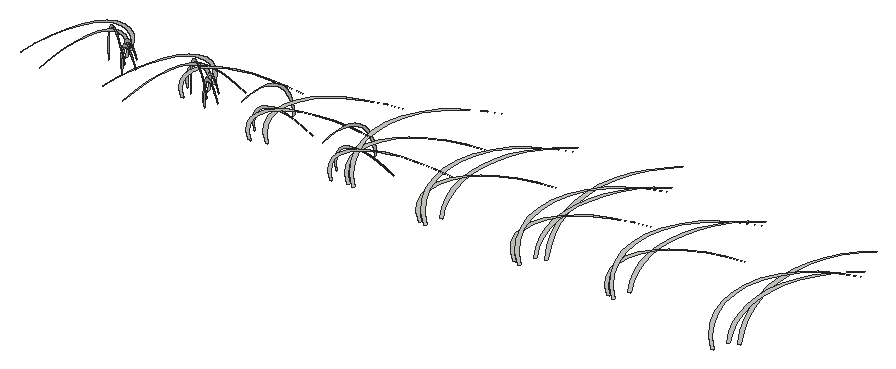
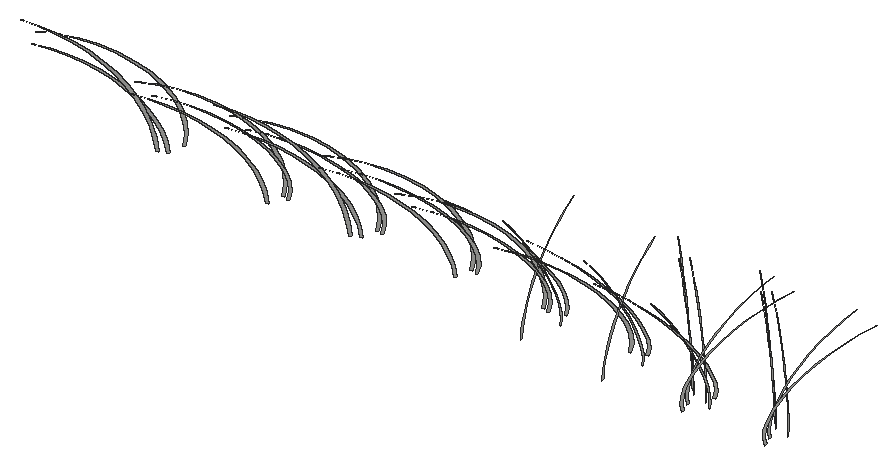
# SketchUp Ruby script. Lengths in inches.
U = 1.inch
M = Sketchup.active_model
def pt(a) = Geom::Point3d.new(a.map { |v| v * U })
def face(e, loops, mat)
  f = e.add_face(loops[0].map { |a| pt(a) })
  loops[1..].each { |l| e.add_face(l.map { |a| pt(a) }).erase! }
  f.material = f.back_material = mat if mat
  f
end
# faces: each face lists its corners as indices into pts; further lists are holes
def faces(e, pts, list, mat = nil) = list.each { |f| face(e, (f[0].is_a?(Array) ? f : [f]).map { |l| l.map { |i| pts[i] } }, mat) }
# xy, xz, yz: faces in a plane at the given z, y or x. An outline is a flat list of corners, or four numbers for a rectangle; further outlines are holes
def ring(l) = l.size == 4 ? [[l[0], l[1]], [l[2], l[1]], [l[2], l[3]], [l[0], l[3]]] : l.each_slice(2).to_a
def flat(e, list, mat, &to3) = list.each { |f| face(e, (f[0].is_a?(Array) ? f : [f]).map { |l| ring(l).map { |u, v| to3.(u, v) } }, mat) }
def xy(e, z, list, mat = nil) = flat(e, list, mat) { |x, y| [x, y, z] }
def xz(e, y, list, mat = nil) = flat(e, list, mat) { |x, z| [x, y, z] }
def yz(e, x, list, mat = nil) = flat(e, list, mat) { |y, z| [x, y, z] }
def lines(e, pts, list) = list.each { |a, b| e.add_line(pt(pts[a]), pt(pts[b])) }
# prism: a flat outline (further loops are holes) pulled along v
def prism(e, loops, v, mat = nil)
  f = face(e, loops, mat); d = Geom::Vector3d.new(v.map { |x| x * U })
  f.pushpull(f.normal.samedirection?(d) ? d.length : -d.length)
end
def box(e, o, s, mat = nil) = prism(e, [[o, [o[0] + s[0], o[1], o[2]], [o[0] + s[0], o[1] + s[1], o[2]], [o[0], o[1] + s[1], o[2]]]], [0, 0, s[2]], mat)
def at(x, y, z, deg = 0) = Geom::Transformation.translation(pt([x, y, z])) * Geom::Transformation.rotation(ORIGIN, Z_AXIS, deg.degrees)
def axes(o, x, y, z) = Geom::Transformation.new([*x, 0, *y, 0, *z, 0, *pt(o).to_a, 1])
def part(name) = M.definitions.add(name)
# library, detail: a bought-in or finely detailed component or shape, given as its bounding box
def library(name, o, s) = part(name).tap { |d| box(d.entities, o, s) }
def detail(e, o, s) = box(e.add_group.entities, o, s)
def put(e, d, t, mat = nil) = e.add_instance(d, t).tap { |i| i.material = mat if mat }
def group(e, t, mat = nil) = e.add_group.tap { |g| g.transformation = t; g.material = mat if mat }.entities
root = M.entities
g1 = group(root,at(402.8125,271.97,0))
p = [[0.125,-0.99,0],[0.06,-0.4375,0],[0,0,1.49],[0.02,-0.18,2.99],[0.12,-0.96,4.45],[0.3,-2.34,5.86],
  [0.54,-4.28,7.16],[0.85,-6.72,8.33],[1.21,-9.61,9.33],[1.62,-12.88,10.15],[2.07,-16.44,10.77],[2.55,-20.21,11.16],
  [3.03,-24.1,11.32],[3.53,-28,11.24],[3.04,-24.17,11.26],[2.57,-20.38,11.05],[2.11,-16.72,10.625],[1.67,-13.27,9.99],
  [1.27,-10.1,9.16],[0.92,-7.3,8.16],[0.62,-4.93,7.01],[0.38,-3.04,5.73],[0.21,-1.67,4.36],[0.11,-0.87,2.93],
  [0.08,-0.64,1.46]]
faces(g1,p,[[0,1,2,3,4,5,6,7,8,9,10,11,12,13,14,15,16,17,18,19,20,21,22,23,24]])
g2 = group(root,at(405.48,266.78,0))
p = [[14.61,-14.77,15.34],[16.8125,-17,15.75],[14.68,-14.84,15.26],[12.62,-12.76,14.58],[10.65,-10.77,13.72],[8.8,-8.9,12.69],
  [7.09,-7.17,11.5],[5.54,-5.61,10.16],[4.17,-4.22,8.7],[2.98,-3.02,7.11],[2,-2.02,5.43],[1.24,-1.25,3.67],
  [0.69,-0.7,1.86],[0.38,-0.38,0],[0,0,0],[0.26,-0.26,1.9],[0.77,-0.77,3.76],[1.52,-1.54,5.57],
  [2.51,-2.53,7.28],[3.72,-3.76,8.9],[5.13,-5.19,10.39],[6.74,-6.8125,11.73],[8.51,-8.61,12.91],[10.43,-10.55,13.91],
  [12.47,-12.61,14.73]]
faces(g2,p,[[0,1,2,3,4,5,6,7,8,9,10,11,12,13,14,15,16,17,18,19,20,21,22,23,24]])
g3 = group(root,at(384.95,272.39,0))
p = [[0.125,-0.99,0],[0.06,-0.4375,0],[0,0,1.49],[0.02,-0.18,2.99],[0.12,-0.96,4.45],[0.3,-2.34,5.86],
  [0.54,-4.28,7.16],[0.85,-6.72,8.33],[1.21,-9.61,9.33],[1.62,-12.88,10.15],[2.07,-16.44,10.77],[2.55,-20.21,11.16],
  [3.03,-24.1,11.32],[3.53,-28,11.24],[3.04,-24.17,11.26],[2.57,-20.38,11.05],[2.11,-16.72,10.625],[1.67,-13.27,9.99],
  [1.27,-10.1,9.16],[0.92,-7.3,8.16],[0.62,-4.93,7.01],[0.38,-3.04,5.73],[0.21,-1.67,4.36],[0.11,-0.87,2.93],
  [0.08,-0.64,1.46]]
faces(g3,p,[[0,1,2,3,4,5,6,7,8,9,10,11,12,13,14,15,16,17,18,19,20,21,22,23,24]])
g4 = group(root,at(387.62,267.2,0))
p = [[14.61,-14.77,15.34],[16.8125,-17,15.75],[14.68,-14.84,15.26],[12.62,-12.76,14.58],[10.65,-10.77,13.72],[8.8,-8.9,12.69],
  [7.09,-7.17,11.5],[5.54,-5.61,10.16],[4.17,-4.22,8.7],[2.98,-3.02,7.11],[2,-2.02,5.43],[1.24,-1.25,3.67],
  [0.69,-0.7,1.86],[0.38,-0.38,0],[0,0,0],[0.26,-0.26,1.9],[0.77,-0.77,3.76],[1.52,-1.54,5.57],
  [2.51,-2.53,7.28],[3.72,-3.76,8.9],[5.13,-5.19,10.39],[6.74,-6.8125,11.73],[8.51,-8.61,12.91],[10.43,-10.55,13.91],
  [12.47,-12.61,14.73]]
faces(g4,p,[[0,1,2,3,4,5,6,7,8,9,10,11,12,13,14,15,16,17,18,19,20,21,22,23,24]])
g5 = group(root,at(436.95,260.375,0))
p = [[0.99,-0.08,0],[0.44,-0.04,0],[0,0,1.49],[0.18,-0.01,2.99],[0.97,-0.08,4.45],[2.35,-0.19,5.86],
  [4.3,-0.35,7.16],[6.75,-0.55,8.33],[9.66,-0.78,9.33],[12.9375,-1.05,10.15],[16.52,-1.34,10.77],[20.31,-1.64,11.16],
  [24.21,-1.96,11.32],[28.13,-2.27,11.24],[24.28,-1.96,11.26],[20.48,-1.66,11.05],[16.8,-1.36,10.625],[13.33,-1.08,9.99],
  [10.15,-0.82,9.16],[7.34,-0.59,8.16],[4.95,-0.4,7.01],[3.05,-0.25,5.73],[1.68,-0.14,4.36],[0.87,-0.07,2.93],
  [0.64,-0.05,1.46]]
faces(g5,p,[[0,1,2,3,4,5,6,7,8,9,10,11,12,13,14,15,16,17,18,19,20,21,22,23,24]])
g6 = group(root,at(435.76,263.67,0))
p = [[0.69,-0.31,0],[0.31,-0.14,0],[0,0,1.24],[0.125,-0.06,2.49],[0.68,-0.3,3.72],[1.65,-0.73,4.89],
  [3.01,-1.34,5.98],[4.73,-2.11,6.95],[6.76,-3.01,7.8],[9.06,-4.04,8.48],[11.5625,-5.15,8.99],[14.21,-6.33,9.32],
  [16.94,-7.55,9.46],[19.6875,-8.77,9.39],[17,-7.58,9.4],[14.33,-6.39,9.23],[11.76,-5.24,8.875],[9.33,-4.16,8.35],
  [7.1,-3.17,7.65],[5.14,-2.29,6.82],[3.47,-1.55,5.86],[2.14,-0.95,4.79],[1.18,-0.52,3.64],[0.61,-0.27,2.45],
  [0.45,-0.2,1.22]]
faces(g6,p,[[0,1,2,3,4,5,6,7,8,9,10,11,12,13,14,15,16,17,18,19,20,21,22,23,24]])
g7 = group(root,at(404.12,268.15,0))
p = [[14.61,-14.77,12.375],[16.8125,-17,12.7],[14.68,-14.84,12.31],[12.62,-12.76,11.76],[10.65,-10.77,11.07],[8.8,-8.9,10.23],
  [7.09,-7.17,9.27],[5.54,-5.61,8.2],[4.17,-4.22,7.01],[2.98,-3.02,5.74],[2,-2.02,4.38],[1.24,-1.25,2.96],
  [0.69,-0.7,1.5],[0.38,-0.38,0],[0,0,0],[0.26,-0.26,1.53],[0.77,-0.77,3.03],[1.52,-1.54,4.49],
  [2.51,-2.53,5.875],[3.72,-3.76,7.18],[5.13,-5.19,8.375],[6.74,-6.8125,9.46],[8.51,-8.61,10.41],[10.43,-10.55,11.22],
  [12.47,-12.61,11.88]]
faces(g7,p,[[0,1,2,3,4,5,6,7,8,9,10,11,12,13,14,15,16,17,18,19,20,21,22,23,24]])
g8 = group(root,at(522.45,254.88,0))
p = [[0.85,0.36,0],[0.38,0.16,0],[0,0,2.37],[0.15,0.0625,4.75],[0.84,0.35,7.08],[2.03,0.85,9.32],
  [3.71,1.54,11.39],[5.83,2.42,13.25],[8.33,3.47,14.85],[11.16,4.65,16.15],[14.25,5.93,17.13],[17.52,7.29,17.75],
  [20.89,8.69,18.01],[24.27,10.1,17.89],[20.95,8.72,17.91],[17.67,7.35,17.58],[14.49,6.03,16.9],[11.5,4.79,15.89],
  [8.76,3.65,14.58],[6.33,2.63,12.99],[4.27,1.78,11.15],[2.63,1.1,9.125],[1.45,0.6,6.94],[0.75,0.3125,4.66],
  [0.55,0.23,2.33]]
faces(g8,p,[[0,1,2,3,4,5,6,7,8,9,10,11,12,13,14,15,16,17,18,19,20,21,22,23,24]])
g9 = group(root,at(400.6,269.28,0))
p = [[0.65,-0.66,0],[0.29,-0.29,0],[0,0,1.75],[0.12,-0.12,3.51],[0.64,-0.64,5.24],[1.55,-1.5625,6.89],
  [2.82,-2.86,8.42],[4.4375,-4.49,9.8],[6.35,-6.42,10.98],[8.5,-8.6,11.95],[10.85,-10.98,12.67],[13.34,-13.49,13.13],
  [15.91,-16.09,13.32],[18.48,-18.69,13.23],[15.96,-16.14,13.25],[13.45,-13.61,13],[11.04,-11.16,12.5],[8.76,-8.86,11.75],
  [6.67,-6.74,10.78],[4.82,-4.875,9.6],[3.25,-3.29,8.25],[2.01,-2.03,6.75],[1.11,-1.12,5.13],[0.57,-0.58,3.44],
  [0.42,-0.42,1.72]]
faces(g9,p,[[0,1,2,3,4,5,6,7,8,9,10,11,12,13,14,15,16,17,18,19,20,21,22,23,24]])
g10 = group(root,at(386.26,268.57,0))
p = [[14.61,-14.77,12.375],[16.8125,-17,12.7],[14.68,-14.84,12.31],[12.62,-12.76,11.76],[10.65,-10.77,11.07],[8.8,-8.9,10.23],
  [7.09,-7.17,9.27],[5.54,-5.61,8.2],[4.17,-4.22,7.01],[2.98,-3.02,5.74],[2,-2.02,4.38],[1.24,-1.25,2.96],
  [0.69,-0.7,1.5],[0.38,-0.38,0],[0,0,0],[0.26,-0.26,1.53],[0.77,-0.77,3.03],[1.52,-1.54,4.49],
  [2.51,-2.53,5.875],[3.72,-3.76,7.18],[5.13,-5.19,8.375],[6.74,-6.8125,9.46],[8.51,-8.61,10.41],[10.43,-10.55,11.22],
  [12.47,-12.61,11.88]]
faces(g10,p,[[0,1,2,3,4,5,6,7,8,9,10,11,12,13,14,15,16,17,18,19,20,21,22,23,24]])
g11 = group(root,at(402.15,274.22,0))
p = [[-0.06,-0.99,0],[-0.03,-0.44,0],[0,0,1.49],[-0.01,-0.18,2.99],[-0.06,-0.97,4.45],[-0.14,-2.36,5.86],
  [-0.26,-4.3,7.16],[-0.4,-6.76,8.33],[-0.58,-9.67,9.33],[-0.77,-12.96,10.15],[-0.99,-16.54,10.77],[-1.22,-20.34,11.16],
  [-1.45,-24.24,11.32],[-1.68,-28.17,11.24],[-1.45,-24.32,11.26],[-1.23,-20.51,11.05],[-1.01,-16.82,10.625],[-0.8,-13.35,9.99],
  [-0.61,-10.16,9.16],[-0.4375,-7.35,8.16],[-0.3,-4.96,7.01],[-0.18,-3.06,5.73],[-0.1,-1.69,4.36],[-0.05,-0.87,2.93],
  [-0.04,-0.64,1.46]]
faces(g11,p,[[0,1,2,3,4,5,6,7,8,9,10,11,12,13,14,15,16,17,18,19,20,21,22,23,24]])
g12 = group(root,at(438.27,271.6,0))
p = [[6.07,-19.87,14.56],[6.99,-22.87,14.94],[6.1,-19.96,14.48],[5.25,-17.16,13.83],[4.43,-14.49,13.02],[3.66,-11.97,12.04],
  [2.95,-9.65,10.91],[2.31,-7.54,9.64],[1.73,-5.67,8.25],[1.24,-4.06,6.75],[0.83,-2.72,5.15],[0.51,-1.68,3.49],
  [0.29,-0.94,1.76],[0.16,-0.52,0],[0,0,0],[0.11,-0.35,1.8],[0.32,-1.04,3.57],[0.63,-2.07,5.28],
  [1.04,-3.41,6.91],[1.55,-5.05,8.44],[2.13,-6.98,9.85],[2.8,-9.16,11.13],[3.54,-11.58,12.25],[4.34,-14.1875,13.2],
  [5.1875,-16.96,13.97]]
faces(g12,p,[[0,1,2,3,4,5,6,7,8,9,10,11,12,13,14,15,16,17,18,19,20,21,22,23,24]])
g13 = group(root,at(478,257.67,0))
p = [[0.91,0.18,0],[0.4,0.08,0],[0,0,1.75],[0.16,0.03,3.51],[0.89,0.17,5.24],[2.16,0.42,6.89],
  [3.94,0.76,8.42],[6.19,1.2,9.8],[8.86,1.72,10.98],[11.87,2.3,11.95],[15.16,2.94,12.67],[18.63,3.61,13.13],
  [22.21,4.31,13.32],[25.81,5.01,13.23],[22.28,4.32,13.25],[18.79,3.64,13],[15.41,2.99,12.5],[12.23,2.37,11.75],
  [9.3125,1.81,10.78],[6.73,1.31,9.6],[4.54,0.88,8.25],[2.8,0.54,6.75],[1.54,0.3,5.13],[0.8,0.16,3.44],
  [0.59,0.11,1.72]]
faces(g13,p,[[0,1,2,3,4,5,6,7,8,9,10,11,12,13,14,15,16,17,18,19,20,21,22,23,24]])
g14 = group(root,at(382.74,269.7,0))
p = [[0.65,-0.66,0],[0.29,-0.29,0],[0,0,1.75],[0.12,-0.12,3.51],[0.64,-0.64,5.24],[1.55,-1.5625,6.89],
  [2.82,-2.86,8.42],[4.4375,-4.49,9.8],[6.35,-6.42,10.98],[8.5,-8.6,11.95],[10.85,-10.98,12.67],[13.34,-13.49,13.13],
  [15.91,-16.09,13.32],[18.48,-18.69,13.23],[15.96,-16.14,13.25],[13.45,-13.61,13],[11.04,-11.16,12.5],[8.76,-8.86,11.75],
  [6.67,-6.74,10.78],[4.82,-4.875,9.6],[3.25,-3.29,8.25],[2.01,-2.03,6.75],[1.11,-1.12,5.13],[0.57,-0.58,3.44],
  [0.42,-0.42,1.72]]
faces(g14,p,[[0,1,2,3,4,5,6,7,8,9,10,11,12,13,14,15,16,17,18,19,20,21,22,23,24]])
g15 = group(root,at(384.29,274.64,0))
p = [[-0.06,-0.99,0],[-0.03,-0.44,0],[0,0,1.49],[-0.01,-0.18,2.99],[-0.06,-0.97,4.45],[-0.14,-2.36,5.86],
  [-0.26,-4.3,7.16],[-0.4,-6.76,8.33],[-0.58,-9.67,9.33],[-0.77,-12.96,10.15],[-0.99,-16.54,10.77],[-1.22,-20.34,11.16],
  [-1.45,-24.24,11.32],[-1.68,-28.17,11.24],[-1.45,-24.32,11.26],[-1.23,-20.51,11.05],[-1.01,-16.82,10.625],[-0.8,-13.35,9.99],
  [-0.61,-10.16,9.16],[-0.4375,-7.35,8.16],[-0.3,-4.96,7.01],[-0.18,-3.06,5.73],[-0.1,-1.69,4.36],[-0.05,-0.87,2.93],
  [-0.04,-0.64,1.46]]
faces(g15,p,[[0,1,2,3,4,5,6,7,8,9,10,11,12,13,14,15,16,17,18,19,20,21,22,23,24]])
g16 = group(root,at(497.48,258.41,0))
p = [[0.91,0.18,0],[0.4,0.08,0],[0,0,1.75],[0.16,0.03,3.51],[0.89,0.17,5.24],[2.16,0.42,6.89],
  [3.94,0.76,8.42],[6.19,1.2,9.8],[8.86,1.72,10.98],[11.87,2.3,11.95],[15.16,2.94,12.67],[18.63,3.61,13.13],
  [22.21,4.31,13.32],[25.81,5.01,13.23],[22.28,4.32,13.25],[18.79,3.64,13],[15.41,2.99,12.5],[12.23,2.37,11.75],
  [9.3125,1.81,10.78],[6.73,1.31,9.6],[4.54,0.88,8.25],[2.8,0.54,6.75],[1.54,0.3,5.13],[0.8,0.16,3.44],
  [0.59,0.11,1.72]]
faces(g16,p,[[0,1,2,3,4,5,6,7,8,9,10,11,12,13,14,15,16,17,18,19,20,21,22,23,24]])
g17 = group(root,at(457.34,258.42,0))
p = [[0.91,0.18,0],[0.4,0.08,0],[0,0,1.75],[0.16,0.03,3.51],[0.89,0.17,5.24],[2.16,0.42,6.89],
  [3.94,0.76,8.42],[6.19,1.2,9.8],[8.86,1.72,10.98],[11.87,2.3,11.95],[15.16,2.94,12.67],[18.63,3.61,13.13],
  [22.21,4.31,13.32],[25.81,5.01,13.23],[22.28,4.32,13.25],[18.79,3.64,13],[15.41,2.99,12.5],[12.23,2.37,11.75],
  [9.3125,1.81,10.78],[6.73,1.31,9.6],[4.54,0.88,8.25],[2.8,0.54,6.75],[1.54,0.3,5.13],[0.8,0.16,3.44],
  [0.59,0.11,1.72]]
faces(g17,p,[[0,1,2,3,4,5,6,7,8,9,10,11,12,13,14,15,16,17,18,19,20,21,22,23,24]])
g18 = group(root,at(417.8,262.59,0))
p = [[0.99,-0.08,0],[0.44,-0.04,0],[0,0,1.49],[0.18,-0.01,2.99],[0.97,-0.08,4.45],[2.35,-0.19,5.86],
  [4.3,-0.35,7.16],[6.75,-0.55,8.33],[9.66,-0.78,9.33],[12.9375,-1.05,10.15],[16.52,-1.34,10.77],[20.31,-1.64,11.16],
  [24.21,-1.96,11.32],[28.13,-2.27,11.24],[24.28,-1.96,11.26],[20.48,-1.66,11.05],[16.8,-1.36,10.625],[13.33,-1.08,9.99],
  [10.15,-0.82,9.16],[7.34,-0.59,8.16],[4.95,-0.4,7.01],[3.05,-0.25,5.73],[1.68,-0.14,4.36],[0.87,-0.07,2.93],
  [0.64,-0.05,1.46]]
faces(g18,p,[[0,1,2,3,4,5,6,7,8,9,10,11,12,13,14,15,16,17,18,19,20,21,22,23,24]])
g19 = group(root,at(416.61,265.89,0))
p = [[0.69,-0.31,0],[0.31,-0.14,0],[0,0,1.24],[0.125,-0.06,2.49],[0.68,-0.3,3.72],[1.65,-0.73,4.89],
  [3.01,-1.34,5.98],[4.73,-2.11,6.95],[6.76,-3.01,7.8],[9.06,-4.04,8.48],[11.5625,-5.15,8.99],[14.21,-6.33,9.32],
  [16.94,-7.55,9.46],[19.6875,-8.77,9.39],[17,-7.58,9.4],[14.33,-6.39,9.23],[11.76,-5.24,8.875],[9.33,-4.16,8.35],
  [7.1,-3.17,7.65],[5.14,-2.29,6.82],[3.47,-1.55,5.86],[2.14,-0.95,4.79],[1.18,-0.52,3.64],[0.61,-0.27,2.45],
  [0.45,-0.2,1.22]]
faces(g19,p,[[0,1,2,3,4,5,6,7,8,9,10,11,12,13,14,15,16,17,18,19,20,21,22,23,24]])
g20 = group(root,at(479.4,257.21,0))
p = [[0.85,0.36,0],[0.38,0.16,0],[0,0,2.37],[0.15,0.0625,4.75],[0.84,0.35,7.08],[2.03,0.85,9.32],
  [3.71,1.54,11.39],[5.83,2.42,13.25],[8.33,3.47,14.85],[11.16,4.65,16.15],[14.25,5.93,17.13],[17.52,7.29,17.75],
  [20.89,8.69,18.01],[24.27,10.1,17.89],[20.95,8.72,17.91],[17.67,7.35,17.58],[14.49,6.03,16.9],[11.5,4.79,15.89],
  [8.76,3.65,14.58],[6.33,2.63,12.99],[4.27,1.78,11.15],[2.63,1.1,9.125],[1.45,0.6,6.94],[0.75,0.3125,4.66],
  [0.55,0.23,2.33]]
faces(g20,p,[[0,1,2,3,4,5,6,7,8,9,10,11,12,13,14,15,16,17,18,19,20,21,22,23,24]])
g21 = group(root,at(419.12,273.81,0))
p = [[6.07,-19.87,14.56],[6.99,-22.87,14.94],[6.1,-19.96,14.48],[5.25,-17.16,13.83],[4.43,-14.49,13.02],[3.66,-11.97,12.04],
  [2.95,-9.65,10.91],[2.31,-7.54,9.64],[1.73,-5.67,8.25],[1.24,-4.06,6.75],[0.83,-2.72,5.15],[0.51,-1.68,3.49],
  [0.29,-0.94,1.76],[0.16,-0.52,0],[0,0,0],[0.11,-0.35,1.8],[0.32,-1.04,3.57],[0.63,-2.07,5.28],
  [1.04,-3.41,6.91],[1.55,-5.05,8.44],[2.13,-6.98,9.85],[2.8,-9.16,11.13],[3.54,-11.58,12.25],[4.34,-14.1875,13.2],
  [5.1875,-16.96,13.97]]
faces(g21,p,[[0,1,2,3,4,5,6,7,8,9,10,11,12,13,14,15,16,17,18,19,20,21,22,23,24]])
g22 = group(root,at(498.875,257.95,0))
p = [[0.85,0.36,0],[0.38,0.16,0],[0,0,2.37],[0.15,0.0625,4.75],[0.84,0.35,7.08],[2.03,0.85,9.32],
  [3.71,1.54,11.39],[5.83,2.42,13.25],[8.33,3.47,14.85],[11.16,4.65,16.15],[14.25,5.93,17.13],[17.52,7.29,17.75],
  [20.89,8.69,18.01],[24.27,10.1,17.89],[20.95,8.72,17.91],[17.67,7.35,17.58],[14.49,6.03,16.9],[11.5,4.79,15.89],
  [8.76,3.65,14.58],[6.33,2.63,12.99],[4.27,1.78,11.15],[2.63,1.1,9.125],[1.45,0.6,6.94],[0.75,0.3125,4.66],
  [0.55,0.23,2.33]]
faces(g22,p,[[0,1,2,3,4,5,6,7,8,9,10,11,12,13,14,15,16,17,18,19,20,21,22,23,24]])
g23 = group(root,at(458.74,257.96,0))
p = [[0.85,0.36,0],[0.38,0.16,0],[0,0,2.37],[0.15,0.0625,4.75],[0.84,0.35,7.08],[2.03,0.85,9.32],
  [3.71,1.54,11.39],[5.83,2.42,13.25],[8.33,3.47,14.85],[11.16,4.65,16.15],[14.25,5.93,17.13],[17.52,7.29,17.75],
  [20.89,8.69,18.01],[24.27,10.1,17.89],[20.95,8.72,17.91],[17.67,7.35,17.58],[14.49,6.03,16.9],[11.5,4.79,15.89],
  [8.76,3.65,14.58],[6.33,2.63,12.99],[4.27,1.78,11.15],[2.63,1.1,9.125],[1.45,0.6,6.94],[0.75,0.3125,4.66],
  [0.55,0.23,2.33]]
faces(g23,p,[[0,1,2,3,4,5,6,7,8,9,10,11,12,13,14,15,16,17,18,19,20,21,22,23,24]])
g24 = group(root,at(523.49,258.46,0))
p = [[19.18,7.98,16.73],[22.08,9.1875,17.17],[19.27,8.02,16.64],[16.57,6.9,15.9],[13.98,5.82,14.96],[11.56,4.8125,13.84],
  [9.32,3.88,12.54],[7.28,3.03,11.08],[5.47,2.28,9.48],[3.92,1.63,7.76],[2.63,1.09,5.92],[1.625,0.68,4.01],
  [0.91,0.38,2.02],[0.5,0.21,0],[0,0,0],[0.34,0.14,2.07],[1.01,0.42,4.1],[1.99,0.83,6.07],
  [3.29,1.37,7.94],[4.88,2.03,9.7],[6.74,2.81,11.33],[8.85,3.68,12.79],[11.18,4.65,14.08],[13.7,5.7,15.17],
  [16.375,6.82,16.0625]]
faces(g24,p,[[0,1,2,3,4,5,6,7,8,9,10,11,12,13,14,15,16,17,18,19,20,21,22,23,24]])
g25 = group(root,at(440.03,261.08,0))
p = [[0.91,0.18,0],[0.4,0.08,0],[0,0,1.75],[0.16,0.03,3.51],[0.89,0.17,5.24],[2.16,0.42,6.89],
  [3.94,0.76,8.42],[6.19,1.2,9.8],[8.86,1.72,10.98],[11.87,2.3,11.95],[15.16,2.94,12.67],[18.63,3.61,13.13],
  [22.21,4.31,13.32],[25.81,5.01,13.23],[22.28,4.32,13.25],[18.79,3.64,13],[15.41,2.99,12.5],[12.23,2.37,11.75],
  [9.3125,1.81,10.78],[6.73,1.31,9.6],[4.54,0.88,8.25],[2.8,0.54,6.75],[1.54,0.3,5.13],[0.8,0.16,3.44],
  [0.59,0.11,1.72]]
faces(g25,p,[[0,1,2,3,4,5,6,7,8,9,10,11,12,13,14,15,16,17,18,19,20,21,22,23,24]])
g26 = group(root,at(525.27,259.2,0))
p = [[19.18,7.98,20.75],[22.08,9.1875,21.3],[19.27,8.02,20.63],[16.57,6.9,19.72],[13.98,5.82,18.55],[11.56,4.8125,17.16],
  [9.32,3.88,15.55],[7.28,3.03,13.74],[5.47,2.28,11.76],[3.92,1.63,9.62],[2.63,1.09,7.35],[1.625,0.68,4.97],
  [0.91,0.38,2.51],[0.5,0.21,0],[0,0,0],[0.34,0.14,2.57],[1.01,0.42,5.09],[1.99,0.83,7.53],
  [3.29,1.37,9.85],[4.88,2.03,12.03],[6.74,2.81,14.04],[8.85,3.68,15.86],[11.18,4.65,17.46],[13.7,5.7,18.82],
  [16.375,6.82,19.92]]
faces(g26,p,[[0,1,2,3,4,5,6,7,8,9,10,11,12,13,14,15,16,17,18,19,20,21,22,23,24]])
g27 = group(root,at(480.44,260.78,0))
p = [[19.18,7.98,16.73],[22.08,9.1875,17.17],[19.27,8.02,16.64],[16.57,6.9,15.9],[13.98,5.82,14.96],[11.56,4.8125,13.84],
  [9.32,3.88,12.54],[7.28,3.03,11.08],[5.47,2.28,9.48],[3.92,1.63,7.76],[2.63,1.09,5.92],[1.625,0.68,4.01],
  [0.91,0.38,2.02],[0.5,0.21,0],[0,0,0],[0.34,0.14,2.07],[1.01,0.42,4.1],[1.99,0.83,6.07],
  [3.29,1.37,7.94],[4.88,2.03,9.7],[6.74,2.81,11.33],[8.85,3.68,12.79],[11.18,4.65,14.08],[13.7,5.7,15.17],
  [16.375,6.82,16.0625]]
faces(g27,p,[[0,1,2,3,4,5,6,7,8,9,10,11,12,13,14,15,16,17,18,19,20,21,22,23,24]])
g28 = group(root,at(441.43,260.62,0))
p = [[0.85,0.36,0],[0.38,0.16,0],[0,0,2.37],[0.15,0.0625,4.75],[0.84,0.35,7.08],[2.03,0.85,9.32],
  [3.71,1.54,11.39],[5.83,2.42,13.25],[8.33,3.47,14.85],[11.16,4.65,16.15],[14.25,5.93,17.13],[17.52,7.29,17.75],
  [20.89,8.69,18.01],[24.27,10.1,17.89],[20.95,8.72,17.91],[17.67,7.35,17.58],[14.49,6.03,16.9],[11.5,4.79,15.89],
  [8.76,3.65,14.58],[6.33,2.63,12.99],[4.27,1.78,11.15],[2.63,1.1,9.125],[1.45,0.6,6.94],[0.75,0.3125,4.66],
  [0.55,0.23,2.33]]
faces(g28,p,[[0,1,2,3,4,5,6,7,8,9,10,11,12,13,14,15,16,17,18,19,20,21,22,23,24]])
g29 = group(root,at(420.88,263.29,0))
p = [[0.91,0.18,0],[0.4,0.08,0],[0,0,1.75],[0.16,0.03,3.51],[0.89,0.17,5.24],[2.16,0.42,6.89],
  [3.94,0.76,8.42],[6.19,1.2,9.8],[8.86,1.72,10.98],[11.87,2.3,11.95],[15.16,2.94,12.67],[18.63,3.61,13.13],
  [22.21,4.31,13.32],[25.81,5.01,13.23],[22.28,4.32,13.25],[18.79,3.64,13],[15.41,2.99,12.5],[12.23,2.37,11.75],
  [9.3125,1.81,10.78],[6.73,1.31,9.6],[4.54,0.88,8.25],[2.8,0.54,6.75],[1.54,0.3,5.13],[0.8,0.16,3.44],
  [0.59,0.11,1.72]]
faces(g29,p,[[0,1,2,3,4,5,6,7,8,9,10,11,12,13,14,15,16,17,18,19,20,21,22,23,24]])
g30 = group(root,at(400.09,266.9375,0))
p = [[0.99,-0.08,0],[0.44,-0.04,0],[0,0,1.49],[0.18,-0.01,2.99],[0.97,-0.08,4.45],[2.35,-0.19,5.86],
  [4.3,-0.35,7.16],[6.75,-0.55,8.33],[9.66,-0.78,9.33],[12.9375,-1.05,10.15],[16.52,-1.34,10.77],[20.31,-1.64,11.16],
  [24.21,-1.96,11.32],[28.13,-2.27,11.24],[24.28,-1.96,11.26],[20.48,-1.66,11.05],[16.8,-1.36,10.625],[13.33,-1.08,9.99],
  [10.15,-0.82,9.16],[7.34,-0.59,8.16],[4.95,-0.4,7.01],[3.05,-0.25,5.73],[1.68,-0.14,4.36],[0.87,-0.07,2.93],
  [0.64,-0.05,1.46]]
faces(g30,p,[[0,1,2,3,4,5,6,7,8,9,10,11,12,13,14,15,16,17,18,19,20,21,22,23,24]])
g31 = group(root,at(398.9,270.24,0))
p = [[0.69,-0.31,0],[0.31,-0.14,0],[0,0,1.24],[0.125,-0.06,2.49],[0.68,-0.3,3.72],[1.65,-0.73,4.89],
  [3.01,-1.34,5.98],[4.73,-2.11,6.95],[6.76,-3.01,7.8],[9.06,-4.04,8.48],[11.5625,-5.15,8.99],[14.21,-6.33,9.32],
  [16.94,-7.55,9.46],[19.6875,-8.77,9.39],[17,-7.58,9.4],[14.33,-6.39,9.23],[11.76,-5.24,8.875],[9.33,-4.16,8.35],
  [7.1,-3.17,7.65],[5.14,-2.29,6.82],[3.47,-1.55,5.86],[2.14,-0.95,4.79],[1.18,-0.52,3.64],[0.61,-0.27,2.45],
  [0.45,-0.2,1.22]]
faces(g31,p,[[0,1,2,3,4,5,6,7,8,9,10,11,12,13,14,15,16,17,18,19,20,21,22,23,24]])
g32 = group(root,at(499.91,261.52,0))
p = [[19.18,7.98,16.73],[22.08,9.1875,17.17],[19.27,8.02,16.64],[16.57,6.9,15.9],[13.98,5.82,14.96],[11.56,4.8125,13.84],
  [9.32,3.88,12.54],[7.28,3.03,11.08],[5.47,2.28,9.48],[3.92,1.63,7.76],[2.63,1.09,5.92],[1.625,0.68,4.01],
  [0.91,0.38,2.02],[0.5,0.21,0],[0,0,0],[0.34,0.14,2.07],[1.01,0.42,4.1],[1.99,0.83,6.07],
  [3.29,1.37,7.94],[4.88,2.03,9.7],[6.74,2.81,11.33],[8.85,3.68,12.79],[11.18,4.65,14.08],[13.7,5.7,15.17],
  [16.375,6.82,16.0625]]
faces(g32,p,[[0,1,2,3,4,5,6,7,8,9,10,11,12,13,14,15,16,17,18,19,20,21,22,23,24]])
g33 = group(root,at(482.22,261.52,0))
p = [[19.18,7.98,20.75],[22.08,9.1875,21.3],[19.27,8.02,20.63],[16.57,6.9,19.72],[13.98,5.82,18.55],[11.56,4.8125,17.16],
  [9.32,3.88,15.55],[7.28,3.03,13.74],[5.47,2.28,11.76],[3.92,1.63,9.62],[2.63,1.09,7.35],[1.625,0.68,4.97],
  [0.91,0.38,2.51],[0.5,0.21,0],[0,0,0],[0.34,0.14,2.57],[1.01,0.42,5.09],[1.99,0.83,7.53],
  [3.29,1.37,9.85],[4.88,2.03,12.03],[6.74,2.81,14.04],[8.85,3.68,15.86],[11.18,4.65,17.46],[13.7,5.7,18.82],
  [16.375,6.82,19.92]]
faces(g33,p,[[0,1,2,3,4,5,6,7,8,9,10,11,12,13,14,15,16,17,18,19,20,21,22,23,24]])
g34 = group(root,at(459.78,261.54,0))
p = [[19.18,7.98,16.73],[22.08,9.1875,17.17],[19.27,8.02,16.64],[16.57,6.9,15.9],[13.98,5.82,14.96],[11.56,4.8125,13.84],
  [9.32,3.88,12.54],[7.28,3.03,11.08],[5.47,2.28,9.48],[3.92,1.63,7.76],[2.63,1.09,5.92],[1.625,0.68,4.01],
  [0.91,0.38,2.02],[0.5,0.21,0],[0,0,0],[0.34,0.14,2.07],[1.01,0.42,4.1],[1.99,0.83,6.07],
  [3.29,1.37,7.94],[4.88,2.03,9.7],[6.74,2.81,11.33],[8.85,3.68,12.79],[11.18,4.65,14.08],[13.7,5.7,15.17],
  [16.375,6.82,16.0625]]
faces(g34,p,[[0,1,2,3,4,5,6,7,8,9,10,11,12,13,14,15,16,17,18,19,20,21,22,23,24]])
